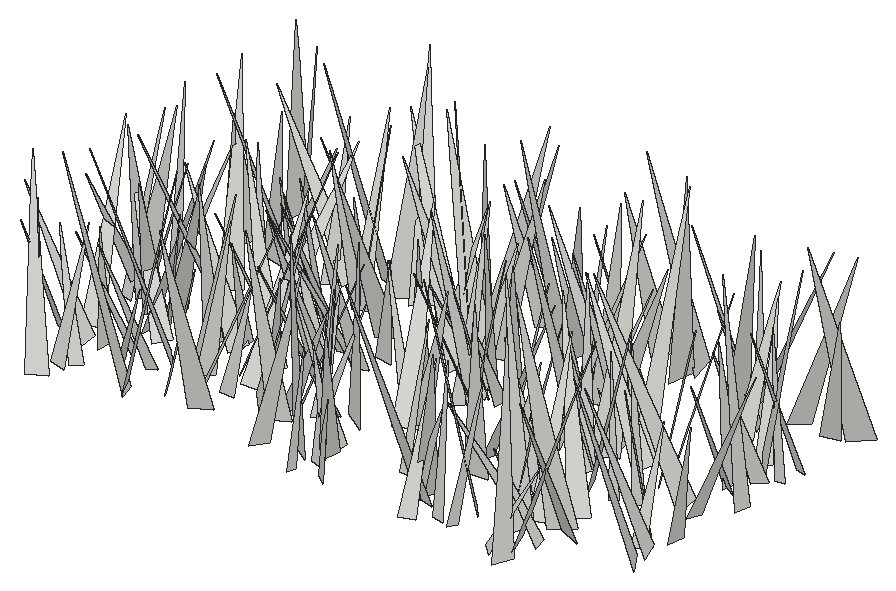
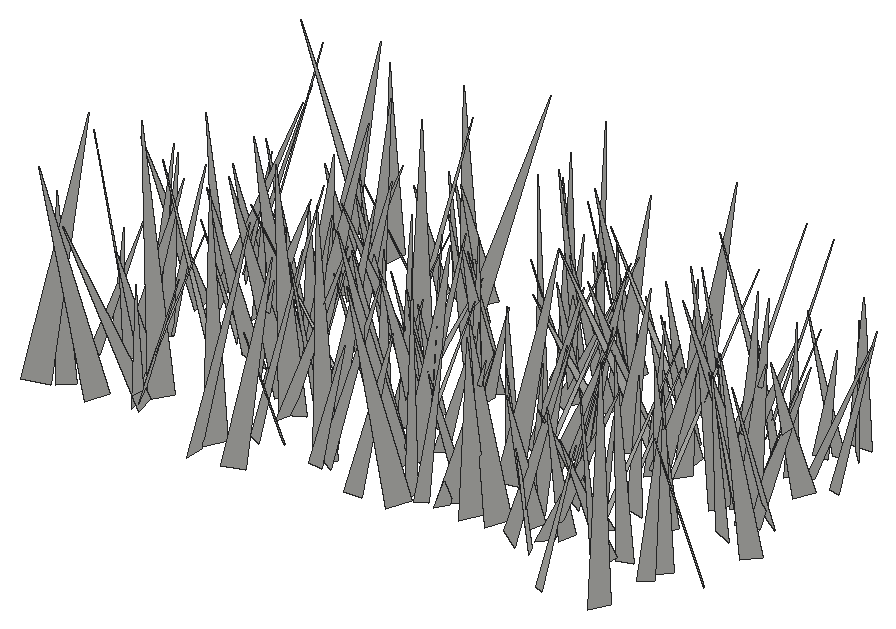
# SketchUp Ruby script. Lengths in inches.
U = 1.inch
M = Sketchup.active_model
def pt(a) = Geom::Point3d.new(a.map { |v| v * U })
def face(e, loops, mat)
  f = e.add_face(loops[0].map { |a| pt(a) })
  loops[1..].each { |l| e.add_face(l.map { |a| pt(a) }).erase! }
  f.material = f.back_material = mat if mat
  f
end
# faces: each face lists its corners as indices into pts; further lists are holes
def faces(e, pts, list, mat = nil) = list.each { |f| face(e, (f[0].is_a?(Array) ? f : [f]).map { |l| l.map { |i| pts[i] } }, mat) }
# xy, xz, yz: faces in a plane at the given z, y or x. An outline is a flat list of corners, or four numbers for a rectangle; further outlines are holes
def ring(l) = l.size == 4 ? [[l[0], l[1]], [l[2], l[1]], [l[2], l[3]], [l[0], l[3]]] : l.each_slice(2).to_a
def flat(e, list, mat, &to3) = list.each { |f| face(e, (f[0].is_a?(Array) ? f : [f]).map { |l| ring(l).map { |u, v| to3.(u, v) } }, mat) }
def xy(e, z, list, mat = nil) = flat(e, list, mat) { |x, y| [x, y, z] }
def xz(e, y, list, mat = nil) = flat(e, list, mat) { |x, z| [x, y, z] }
def yz(e, x, list, mat = nil) = flat(e, list, mat) { |y, z| [x, y, z] }
def lines(e, pts, list) = list.each { |a, b| e.add_line(pt(pts[a]), pt(pts[b])) }
# prism: a flat outline (further loops are holes) pulled along v
def prism(e, loops, v, mat = nil)
  f = face(e, loops, mat); d = Geom::Vector3d.new(v.map { |x| x * U })
  f.pushpull(f.normal.samedirection?(d) ? d.length : -d.length)
end
def box(e, o, s, mat = nil) = prism(e, [[o, [o[0] + s[0], o[1], o[2]], [o[0] + s[0], o[1] + s[1], o[2]], [o[0], o[1] + s[1], o[2]]]], [0, 0, s[2]], mat)
def at(x, y, z, deg = 0) = Geom::Transformation.translation(pt([x, y, z])) * Geom::Transformation.rotation(ORIGIN, Z_AXIS, deg.degrees)
def axes(o, x, y, z) = Geom::Transformation.new([*x, 0, *y, 0, *z, 0, *pt(o).to_a, 1])
def part(name) = M.definitions.add(name)
# library, detail: a bought-in or finely detailed component or shape, given as its bounding box
def library(name, o, s) = part(name).tap { |d| box(d.entities, o, s) }
def detail(e, o, s) = box(e.add_group.entities, o, s)
def put(e, d, t, mat = nil) = e.add_instance(d, t).tap { |i| i.material = mat if mat }
def group(e, t, mat = nil) = e.add_group.tap { |g| g.transformation = t; g.material = mat if mat }.entities
root = M.entities
c1 = part("fur_instance\#9")
p = [[0.8125,0,1.79],[0.67,-0.02,1.48],[0,-0.11,0],[0,0.11,0]]
faces(c1.entities,p,[[0,1,2,3]])
put(root,c1,axes([541.56,330.53,-21.66],[-6.82221,1.72842,2.33339],[1.55801,7.20655,-0.7829],[2.45045,0.23004,6.99407]))
put(root,c1,axes([539.97,331.04,-21.66],[2.36408,2.77163,0.06713],[2.67068,-2.25294,-1.03299],[0.74428,-0.71945,3.49339]))
put(root,c1,axes([533.52,333.23,-21.66],[-2.92587,-7.18113,1.16279],[-7.26033,2.80394,-0.95233],[-0.45638,1.43204,7.69561]))
put(root,c1,axes([533.1875,333.78,-21.66],[6.03142,-3.81553,0.06105],[-3.78285,-5.99326,-0.84318],[-0.50203,-0.68018,7.08699]))
put(root,c1,axes([516.45,333.74,-21.66],[2.5513,-6.67742,1.15565],[-6.68995,-2.67869,-0.70836],[-1.08074,0.81812,7.11304]))
put(root,c1,axes([525.87,333.9375,-21.66],[5.72206,-2.67718,0.30846],[-2.55509,-5.6197,-1.37653],[-0.85672,-1.12072,6.16558]))
put(root,c1,axes([525.14,331.34,-21.66],[-3.53887,0.08812,1.47041],[-0.2173,3.75324,-0.74791],[1.45693,0.77383,3.46005]))
put(root,c1,axes([541.94,333.51,-21.66],[-3.71284,-0.24914,0.82183],[0.046,3.58403,1.29433],[0.85753,-1.27095,3.48884]))
put(root,c1,axes([527.2,331.49,-21.66],[3.68214,4.39884,2.0354],[4.4735,-4.06815,0.69917],[-1.86561,-1.07294,5.69378]))
put(root,c1,axes([542.73,335.26,-21.66],[-1.67702,-6.45132,0.05531],[-6.32349,1.655,1.30744],[1.27907,-0.27646,6.53625]))
put(root,c1,axes([532.82,333.23,-21.66],[2.13927,-3.81253,0.27989],[-3.71667,-1.99926,1.17453],[0.89447,0.81104,4.21098]))
put(root,c1,axes([524.15,333.3,-21.66],[3.79237,5.90894,3.79832],[6.9076,-3.92109,-0.79686],[-1.27587,-3.6653,6.97586]))
put(root,c1,axes([533.98,331.07,-21.66],[-3.10832,3.75001,0.92239],[3.63037,3.24121,-0.94342],[1.31674,-0.08395,4.77852]))
put(root,c1,axes([506.01,331.8,-21.66],[2.91004,3.86675,2.0314],[3.84438,-3.42612,1.0144],[-2.0734,-0.92551,4.73192]))
put(root,c1,axes([506.5,330.92,-21.66],[-2.09458,6.39775,0.76013],[6.40195,1.97698,1.00139],[-0.72385,-1.02792,6.657]))
put(root,c1,axes([511.85,332.63,-21.66],[-7.0839,-2.86843,1.00142],[-2.98784,7.03787,-0.97651],[0.55097,1.28563,7.57997]))
put(root,c1,axes([540.91,332.69,-21.66],[7.89024,2.57718,0.73013],[2.64489,-7.85516,-0.85554],[-0.42369,-1.04189,8.25626]))
put(root,c1,axes([535.51,332.02,-21.66],[1.56469,4.5597,1.40699],[4.65343,-1.78584,0.61247],[-1.05645,-1.11294,4.78163]))
put(root,c1,axes([521.78,332.56,-21.66],[5.79665,-1.91222,1.6292],[-2.17494,-5.87047,0.84811],[-1.25719,1.33905,6.04471]))
put(root,c1,axes([506.71,332.58,-21.66],[0.82444,4.69785,1.50621],[4.90559,-0.61872,-0.75536],[0.52313,-1.60174,4.70945]))
put(root,c1,axes([536.58,332.05,-21.66],[-4.01234,0.85775,1.7856],[0.34464,4.27421,-1.27879],[1.95072,1.00913,3.89863]))
put(root,c1,axes([547.68,335.24,-21.66],[-5.81163,-3.8947,1.27527],[-3.71182,5.94036,1.22659],[1.73708,-0.33677,6.88761]))
put(root,c1,axes([525.62,334.3,-21.66],[3.23004,-2.47849,1.2151],[-2.38486,-3.44753,-0.69249],[-1.3899,0.15559,4.01205]))
put(root,c1,axes([513.48,334.33,-21.66],[4.61843,1.91697,0.98697],[2.11588,-4.47821,-1.2031],[-0.41467,-1.49987,4.85358]))
put(root,c1,axes([507.57,333.29,-21.66],[-1.66438,3.94539,0.96796],[4.04045,1.49913,0.83702],[-0.42169,-1.20819,4.19948]))
put(root,c1,axes([526.01,332.76,-21.66],[2.58836,6.22661,1.98748],[6.38761,-2.86286,0.6503],[-1.38536,-1.56644,6.71174]))
put(root,c1,axes([511.66,332.62,-21.66],[6.24718,3.3719,1.68528],[3.2403,-6.4703,0.93425],[-1.92623,0.05148,7.03734]))
put(root,c1,axes([504.36,336,-21.66],[-1.82022,-4.66244,0.24993],[-4.60062,1.83672,0.75812],[0.79693,-0.04591,4.9474]))
put(root,c1,axes([536.6875,334.27,-21.66],[-5.72763,-4.55632,1.57593],[-4.80185,5.61014,-1.23206],[0.43111,1.95337,7.21442]))
put(root,c1,axes([509.44,335.03,-21.66],[3.62629,-0.3933,0.08931],[-0.3696,-3.56406,-0.68808],[-0.16141,-0.67481,3.58206]))
put(root,c1,axes([520.99,335.46,-21.66],[1.6386,-6.2759,2.07036],[-6.47654,-1.94928,-0.78297],[-1.31443,1.78093,6.43885]))
put(root,c1,axes([541.84,335.72,-21.66],[2.92408,-7.38877,2.72238],[-7.56214,-3.44459,-1.22649],[-2.19528,2.02396,7.85111]))
put(root,c1,axes([511.32,335.62,-21.66],[-0.67131,-4.1889,0.93111],[-4.10147,0.34927,-1.38579],[-1.26165,1.09345,4.00962]))
put(root,c1,axes([547.5,336.76,-21.66],[-5.8236,-1.97497,1.08531],[-1.72724,5.8434,1.36532],[1.44743,-0.9731,5.99589]))
put(root,c1,axes([509.05,336.7,-21.66],[-4.05728,-2.523,0.42943],[-2.40041,4.03064,1.00168],[0.88766,-0.63233,4.67158]))
put(root,c1,axes([511.47,337.29,-21.66],[-5.81753,-5.50464,0.89808],[-5.45533,5.88597,0.73893],[1.16061,0.07452,7.97488]))
put(root,c1,axes([507.45,336.1,-21.66],[4.3427,-1.50818,1.19732],[-1.3579,-4.49272,-0.73402],[-1.36538,-0.32877,4.53816]))
put(root,c1,axes([540.08,334.25,-21.66],[-7.50799,1.69583,1.59774],[1.55933,7.66276,-0.80567],[1.73121,0.45255,7.65484]))
put(root,c1,axes([506.3,335.9375,-21.66],[-5.398,0.07669,0.31538],[0.11355,5.36878,0.63804],[0.30406,-0.64352,5.36071]))
put(root,c1,axes([525.82,335.21,-21.66],[-5.12979,-1.0122,0.11272],[-1.018,5.07872,-0.72273],[-0.03042,0.73083,5.17851]))
put(root,c1,axes([538.33,335.78,-21.66],[3.90059,1.73334,0.99556],[1.91928,-3.85762,-0.80331],[-0.55855,-1.15086,4.19211]))
put(root,c1,axes([516.6,335.97,-21.66],[-0.37702,3.57753,2.02822],[3.88687,0.97529,-0.99777],[1.34335,-1.81786,3.4562]))
put(root,c1,axes([520.51,336.86,-21.66],[3.4493,-3.36014,0.02886],[-3.29462,-3.37365,0.97621],[0.66096,0.719,4.71542]))
put(root,c1,axes([535.66,337.69,-21.66],[-3.34335,-1.51871,0.13226],[-1.40215,3.18862,1.16988],[0.59829,-1.01398,3.48078]))
put(root,c1,axes([533.93,337.52,-21.66],[1.85268,-6.56464,1.39244],[-6.70428,-1.74747,0.68181],[0.2934,1.52239,6.78691]))
put(root,c1,axes([518.4,337.87,-21.66],[5.40312,-1.02873,0.51523],[-0.87968,-5.28821,-1.33359],[-0.74156,-1.2223,5.33606]))
put(root,c1,axes([514.91,335.92,-21.66],[6.15209,3.35933,0.33959],[3.37614,-6.1107,-0.71393],[0.04606,-0.78923,6.97306]))
put(root,c1,axes([523.08,338.05,-21.66],[-1.88046,-5.21634,0.33238],[-5.10911,1.75978,-1.28722],[-1.10347,0.74146,5.39346]))
put(root,c1,axes([518.49,336.52,-21.66],[5.36031,4.39922,1.5205],[4.6383,-5.24227,-1.18439],[-0.38885,-1.88772,6.83252]))
put(root,c1,axes([530.55,335.12,-21.66],[1.48106,4.37962,0.44895],[4.22706,-1.54701,1.14671],[-1.23071,-0.04293,4.4788]))
put(root,c1,axes([524.4,338.14,-21.66],[-2.31612,-6.1908,2.36322],[-6.27799,2.85121,1.3163],[2.12077,1.67923,6.47748]))
put(root,c1,axes([522.84,336.87,-21.66],[2.35379,3.88662,0.95748],[3.9563,-2.09005,-1.24191],[0.60851,-1.44527,4.3708]))
put(root,c1,axes([514.25,337.01,-21.66],[4.29417,-2.87763,1.75823],[-3.19183,-4.38696,0.6155],[-1.08829,1.5119,5.13243]))
put(root,c1,axes([540.23,335.51,-21.66],[-3.17134,4.85922,0.78552],[4.77597,3.26378,-0.90795],[1.19131,-0.14895,5.73106]))
put(root,c1,axes([546.72,336.72,-21.66],[-2.21972,3.26489,1.22418],[3.2229,2.47495,-0.75684],[1.3308,-0.54808,3.87477]))
put(root,c1,axes([547.09,337.51,-21.66],[2.56501,3.25674,2.5986],[3.3721,-3.41499,0.95138],[-2.44704,-1.29222,4.03491]))
put(root,c1,axes([547.91,338.72,-21.66],[4.83385,-1.43847,0.54232],[-1.36908,-4.84202,-0.64023],[-0.69925,-0.46374,5.00254]))
put(root,c1,axes([522.52,337.2,-21.66],[-2.57998,2.99071,1.64125],[3.02202,2.95835,-0.64026],[1.58287,-0.77341,3.89753]))
put(root,c1,axes([538,338.5625,-21.66],[-4.52682,2.09063,1.69581],[2.46981,4.54531,0.98938],[1.07078,-1.64562,4.88712]))
put(root,c1,axes([535.84,337.99,-21.66],[1.71183,-4.04593,1.56999],[-4.29437,-1.33542,1.2409],[0.62675,1.9005,4.21427]))
put(root,c1,axes([507.27,340.95,-21.66],[4.70982,-4.44224,0.12242],[-4.38661,-4.67586,-0.90827],[-0.71149,-0.57769,6.41023]))
put(root,c1,axes([541.74,337.39,-21.66],[-2.77056,6.19265,0.76015],[6.19361,2.62958,1.15202],[-0.75223,-1.15721,6.68563]))
put(root,c1,axes([512.31,340.11,-21.66],[5.42089,-2.3865,1.81758],[-2.19868,-5.71457,-0.94576],[-2.04078,-0.18248,5.84696]))
put(root,c1,axes([521.05,337.22,-21.66],[4.24517,2.47398,0.29086],[2.34061,-4.15824,1.20716],[-0.85248,0.90284,4.76286]))
put(root,c1,axes([512.71,338.43,-21.66],[5.08359,-0.28901,1.82683],[-0.68576,-5.25683,1.07667],[-1.71772,1.24337,4.97667]))
put(root,c1,axes([527.8,339.99,-21.66],[3.51302,-4.23345,1.0034],[-4.35037,-3.40123,0.88101],[0.05668,1.33409,5.43021]))
put(root,c1,axes([509.77,338.5625,-21.66],[-3.53792,4.34861,0.23075],[4.30519,3.44804,1.02808],[-0.65501,-0.82532,5.51093]))
put(root,c1,axes([517.29,337.51,-21.66],[-1.69129,6.09931,0.73665],[6.01995,1.79783,-1.06428],[1.22654,-0.41345,6.23934]))
put(root,c1,axes([513.87,341.21,-21.66],[4.34393,-1.36952,0.92271],[-1.07858,-4.31928,-1.3331],[-1.25046,-1.03195,4.35524]))
put(root,c1,axes([508.99,340.11,-21.66],[3.83115,1.46002,1.29175],[1.69697,-3.89964,-0.62537],[-0.95945,-1.06731,4.05194]))
put(root,c1,axes([512.04,342.14,-21.66],[-5.96811,-4.81477,0.42538],[-4.75156,5.96808,0.88657],[0.88638,-0.42578,7.61672]))
put(root,c1,axes([505.45,337.41,-21.66],[-4.47188,4.60163,0.40246],[4.4512,4.44255,-1.33612],[1.23441,0.65071,6.27595]))
put(root,c1,axes([508.34,341.62,-21.66],[6.88515,-2.28469,0.18682],[-2.24647,-6.84269,-0.88939],[-0.45618,-0.78602,7.19959]))
put(root,c1,axes([505.62,342.13,-21.66],[0.74185,-5.118,0.35857],[-5.01336,-0.80012,-1.04825],[-1.09027,0.19676,5.06413]))
put(root,c1,axes([508.27,339.13,-21.66],[6.55283,1.12937,1.12544],[0.97488,-6.60494,0.95181],[-1.26162,0.76214,6.58096]))
put(root,c1,axes([518.27,342.4,-21.66],[1.50349,-5.86365,0.5049],[-5.82358,-1.55753,-0.74685],[-0.85041,0.2992,6.00709]))
put(root,c1,axes([540.07,340.5,-21.66],[5.73054,2.09287,1.0832],[2.24178,-5.71944,-0.8093],[-0.7265,-1.14039,6.04684]))
put(root,c1,axes([513.75,340.67,-21.66],[-5.32926,2.77314,1.19327],[2.9808,5.21718,1.1879],[0.47858,-1.6143,5.88899]))
put(root,c1,axes([505.83,342.23,-21.66],[4.78165,-4.93816,1.39024],[-4.88475,-4.96331,-0.82896],[-1.56762,0.40313,6.82367]))
put(root,c1,axes([533.17,339.55,-21.66],[5.62442,0.34622,0.61815],[0.22701,-5.5658,1.05184],[-0.67115,1.01884,5.53603]))
put(root,c1,axes([515.5625,338.77,-21.66],[6.75975,3.62956,0.52461],[3.54067,-6.74583,1.04905],[-0.95528,0.68056,7.60048]))
put(root,c1,axes([519.79,343.73,-21.66],[-4.86076,-4.47494,0.06756],[-4.36579,4.76306,1.38194],[0.98465,-0.972,6.46083]))
put(root,c1,axes([516.86,340.05,-21.66],[-4.60264,5.20733,0.96805],[5.29634,4.53648,0.77902],[0.04773,-1.24166,6.90606]))
put(root,c1,axes([545.83,342.34,-21.66],[-8.03194,-0.35365,0.82088],[-0.22203,7.97883,1.26494],[0.86581,-1.23463,7.93959]))
put(root,c1,axes([538.1,342.38,-21.66],[-1.48143,-7.59825,2.03928],[-7.84224,1.26126,-0.99758],[-0.62555,2.18232,7.67677]))
put(root,c1,axes([526.82,340.23,-21.66],[-4.67353,1.04438,0.03845],[1.02272,4.60667,-0.8165],[0.21505,0.78861,4.71868]))
put(root,c1,axes([543.59,340.64,-21.66],[-4.82421,0.67017,1.12309],[0.52178,4.9221,-0.69578],[1.19925,0.5543,4.82058]))
put(root,c1,axes([542.04,340.23,-21.66],[0.68638,4.30492,0.85677],[4.11958,-0.93113,1.37825],[-1.51508,-0.58153,4.13569]))
put(root,c1,axes([527.17,339.36,-21.66],[-3.85678,5.81728,0.33644],[5.7739,3.8696,-0.71896],[0.78484,0.11882,6.94252]))
put(root,c1,axes([530.33,342.53,-21.66],[-3.6362,-3.51378,0.23491],[-3.4583,3.49912,-1.19165],[-0.6648,1.01649,4.91412]))
put(root,c1,axes([520.81,343.1875,-21.66],[-0.18696,-5.47828,1.21386],[-5.53827,-0.01495,-0.92048],[-0.90141,1.22808,5.40363]))
put(root,c1,axes([546.94,341.67,-21.66],[5.55155,-0.72144,0.45458],[-0.77671,-5.51397,0.73462],[-0.35191,0.78896,5.54982]))
put(root,c1,axes([513.29,344.1,-21.66],[-3.4189,-2.83051,0.24342],[-2.77437,3.40847,0.66713],[0.61145,-0.36118,4.38812]))
put(root,c1,axes([537.24,344.0625,-21.66],[4.28198,-1.79299,1.3249],[-1.43721,-4.41332,-1.32759],[-1.70429,-0.78312,4.44833]))
put(root,c1,axes([537.33,342.74,-21.66],[-3.51582,-2.14374,0.80605],[-2.26912,3.46073,-0.69338],[0.31056,1.01688,4.05904]))
put(root,c1,axes([524.47,344.43,-21.66],[-0.27546,-6.0552,1.07535],[-6.00995,0.49341,1.23885],[1.30474,0.99438,5.93351]))
put(root,c1,axes([538.68,341.87,-21.66],[-5.6137,1.8249,1.28834],[1.63706,5.7317,-0.98561],[1.51991,0.56669,5.82001]))
put(root,c1,axes([517.29,343.69,-21.66],[-3.50463,1.38607,1.3282],[1.66931,3.56562,0.68373],[0.94799,-1.15452,3.70623]))
put(root,c1,axes([504.88,341.3,-21.66],[2.36342,5.34352,0.74133],[5.25737,-2.46286,0.99138],[-1.20944,-0.26392,5.75813]))
put(root,c1,axes([504.83,343.83,-21.66],[4.88196,1.64498,0.71636],[1.77456,-4.73338,-1.22423],[-0.26474,-1.39349,5.00407]))
put(root,c1,axes([546.35,345.47,-21.66],[-1.70648,-4.83175,0.15849],[-4.67215,1.69151,1.26205],[1.24174,-0.27565,4.96639]))
put(root,c1,axes([518.73,344.09,-21.66],[-1.8038,-4.78632,0.84713],[-4.75617,1.55162,-1.36069],[-1.00264,1.25053,4.93062]))
put(root,c1,axes([529.75,345.1,-21.66],[2.79879,-2.29313,0.37979],[-2.08936,-2.74248,-1.16161],[-1.01846,-0.6755,3.42672]))
put(root,c1,axes([533.73,342.74,-21.66],[3.61402,1.40651,0.81578],[1.29809,-3.69316,0.61679],[-0.97915,0.29527,3.8287]))
put(root,c1,axes([528.375,344.39,-21.66],[-6.31827,-0.38458,1.65434],[-0.20418,6.49842,0.73085],[1.68614,-0.65417,6.28763]))
put(root,c1,axes([521.23,344.8125,-21.66],[0.93641,-4.49496,0.58968],[-4.44892,-0.79539,1.00188],[0.87152,0.76939,4.48082]))
put(root,c1,axes([529.68,342.41,-21.66],[4.20978,2.5999,1.29958],[2.36123,-4.39284,1.13935],[-1.69498,0.33775,4.81493]))
put(root,c1,axes([528.42,345.37,-21.66],[-1.9531,-3.93926,0.49775],[-3.87343,2.01224,0.72636],[0.87298,0.11511,4.33645]))
put(root,c1,axes([516.32,345.5,-21.66],[-3.7934,-3.57067,0.95546],[-3.47781,3.9116,0.81037],[1.25196,0.04698,5.14615]))
put(root,c1,axes([541.03,344.29,-21.66],[-5.49496,2.98551,0.84144],[3.09795,5.36781,1.18541],[0.15494,-1.44541,6.14025]))
put(root,c1,axes([528.74,345.63,-21.66],[-1.97091,-5.99186,1.73382],[-5.97714,2.33419,1.27215],[1.7839,1.20092,6.17807]))
put(root,c1,axes([519.7,347.12,-21.66],[2.52782,-6.77606,0.30453],[-6.73549,-2.54598,-0.74076],[-0.80053,0.02468,7.19418]))
put(root,c1,axes([527.9,343.41,-21.66],[3.76541,-0.98312,2.37268],[-1.72485,-4.08783,1.04352],[-1.9029,1.75998,3.74912]))
put(root,c1,axes([503.2,345.1875,-21.66],[2.93008,-5.46925,1.49234],[-5.65269,-2.69042,1.23848],[0.43226,1.89052,6.07982]))
put(root,c1,axes([546.32,345.91,-21.66],[5.03393,-2.19184,1.50174],[-1.99616,-5.24318,-0.96135],[-1.75349,-0.32355,5.40559]))
put(root,c1,axes([543.01,343.3,-21.66],[3.77893,2.89431,1.05154],[2.64296,-3.90266,1.24382],[-1.58036,0.3941,4.59459]))
put(root,c1,axes([538.375,346.19,-21.66],[-6.39849,-1.36399,1.46981],[-1.16574,6.52941,0.98452],[1.63152,-0.68393,6.46776]))
put(root,c1,axes([526.34,347.17,-21.66],[-3.05725,-3.63504,0.09512],[-3.51202,2.98398,1.15363],[0.94245,-0.67208,4.60753]))
put(root,c1,axes([548.6,344.05,-21.66],[-7.01031,-0.43579,1.43561],[-0.72042,6.99511,-1.39453],[1.31601,1.50792,6.88401]))
put(root,c1,axes([506.15,344.17,-21.66],[1.54209,5.92638,1.72605],[6.04197,-1.81335,0.82809],[-1.2633,-1.43843,6.06748]))
put(root,c1,axes([538.4,343.94,-21.66],[-4.94866,6.16749,2.69055],[6.18584,5.48419,-1.19385],[2.6481,-1.28527,7.81677]))
put(root,c1,axes([528.09,344.72,-21.66],[-2.58112,4.19595,2.18678],[4.13957,3.20902,-1.27135],[2.29171,-1.07069,4.75939]))
put(root,c1,axes([547.41,347.16,-21.66],[1.87791,-4.76016,0.94457],[-4.63856,-2.05833,-1.15104],[-1.42657,0.4266,4.98606]))
put(root,c1,axes([528.99,347.16,-21.66],[4.92449,-2.5321,0.51516],[-2.43841,-4.92066,-0.87679],[-0.85503,-0.55051,5.46748]))
put(root,c1,axes([522.125,346.92,-21.66],[0.84886,-4.32385,0.54485],[-4.30912,-0.7498,0.76315],[0.65118,0.6747,4.3398]))
put(root,c1,axes([511.91,345.19,-21.66],[-0.00345,4.9845,1.60202],[5.18158,-0.22632,0.71534],[-0.75028,-1.58596,4.93291]))
put(root,c1,axes([535.35,343.38,-21.66],[4.61833,5.37447,0.17353],[5.34108,-4.61135,0.67253],[-0.62281,0.30742,7.05419]))
put(root,c1,axes([527.52,344.41,-21.66],[0.92539,5.82013,0.73982],[5.78512,-1.02986,0.86568],[-0.97656,-0.58571,5.82931]))
put(root,c1,axes([530.06,346.56,-21.66],[3.37975,2.64749,1.02841],[2.82915,-3.2791,-0.85611],[-0.25046,-1.31446,4.20701]))
put(root,c1,axes([539.36,346.29,-21.66],[-2.08975,2.94897,0.92989],[3.09202,1.98432,0.65582],[-0.0238,-1.13764,3.55435]))
put(root,c1,axes([525.2,346.6,-21.66],[-3.9914,1.89648,0.82188],[2.01712,3.964,0.64912],[0.45094,-0.94526,4.3711]))
put(root,c1,axes([536.39,346.9,-21.66],[5.35038,-4.23141,0.69897],[-4.27634,-5.17862,1.38378],[0.32603,1.51562,6.67957]))
put(root,c1,axes([513.27,346.45,-21.66],[-1.82115,-3.36265,1.61921],[-3.73204,1.65736,-0.7556],[0.03439,1.7865,3.74875]))
put(root,c1,axes([515.16,346.69,-21.66],[-1.86227,-3.58892,1.59018],[-3.91628,1.57852,-1.02377],[-0.26793,1.87217,3.91156]))
put(root,c1,axes([541.4375,347.21,-21.66],[5.88028,2.97965,0.94292],[3.11911,-5.72141,-1.37172],[-0.19635,-1.65292,6.44782]))
put(root,c1,axes([511.94,348.58,-21.66],[-5.99234,-4.15881,0.58341],[-4.19764,5.96205,-0.6148],[0.12593,0.83815,7.26814]))
put(root,c1,axes([509.05,345.8,-21.66],[-5.83364,4.02968,1.05878],[3.90844,5.92385,-1.01134],[1.44341,0.24573,7.01761]))
put(root,c1,axes([534.62,348.62,-21.66],[2.7668,-7.06079,2.0724],[-7.35623,-2.5972,0.97226],[0.18857,2.28135,7.52095]))
put(root,c1,axes([516.43,348.72,-21.66],[0.40641,-5.35004,1.66525],[-5.54368,-0.62666,-0.66032],[-0.81458,1.59547,5.32467]))
put(root,c1,axes([516.32,349.23,-21.66],[4.42301,-0.66017,1.25029],[-0.31732,-4.46498,-1.23502],[-1.37781,-1.09094,4.29808]))
put(root,c1,axes([540.4,344.97,-21.66],[0.71123,8.26754,0.30404],[8.18462,-0.74766,1.1847],[-1.20692,-0.19821,8.21307]))
put(root,c1,axes([523.04,347.84,-21.66],[2.00403,4.77087,1.2081],[4.88814,-1.77806,-1.08691],[0.57161,-1.52123,5.05925]))
put(root,c1,axes([534.01,347.0625,-21.66],[2.59525,5.12132,1.23508],[5.09738,-2.78884,0.85303],[-1.33041,-0.69505,5.67763]))
put(root,c1,axes([506.05,349.76,-21.66],[5.02867,-2.50397,0.95955],[-2.41233,-5.11484,-0.70513],[-1.17101,-0.21602,5.57317]))
put(root,c1,axes([534.87,349.08,-21.66],[-6.53044,0.59698,0.86107],[0.69842,6.53195,0.76827],[0.78105,-0.84949,6.51251]))
put(root,c1,axes([525.59,348.375,-21.66],[-4.55755,6.1935,2.40469],[6.62517,4.45559,1.08074],[0.49905,-2.58872,7.61332]))
put(root,c1,axes([524.87,348.28,-21.66],[-5.85102,-5.01294,3.05498],[-5.59861,6.06235,-0.77491],[1.76582,2.61061,7.66574]))
put(root,c1,axes([546.52,348.53,-21.66],[-3.91032,-4.73518,3.93684],[-5.20514,5.03349,0.88414],[3.29046,2.33522,6.07707]))
put(root,c1,axes([548.22,347.98,-21.66],[0.93593,4.40998,1.37185],[4.37962,-1.29175,1.16453],[-1.46587,-1.0437,4.3552]))
put(root,c1,axes([548.48,349.64,-21.66],[-2.25031,-4.2676,0.76277],[-4.32128,2.13921,-0.77999],[-0.34742,1.03417,4.76108]))
put(root,c1,axes([508.67,350.09,-21.66],[0.4901,-6.09421,1.40714],[-6.12992,-0.18765,1.32232],[1.24239,1.47818,5.96918]))
put(root,c1,axes([530.84,350.21,-21.66],[-1.51779,-7.89387,2.17922],[-8.18213,1.37007,-0.73587],[-0.33897,2.275,8.00471]))
put(root,c1,axes([526.27,349.11,-21.66],[4.89354,-4.52263,1.72188],[-4.82903,-4.72322,1.31813],[-0.31551,2.14541,6.53173]))
put(root,c1,axes([529.74,351.7,-21.66],[6.8807,-3.2851,0.24825],[-3.20439,-6.80705,-1.26238],[-0.76512,-1.03432,7.51946]))
put(root,c1,axes([503.4,349.42,-21.66],[3.56732,3.05528,0.6125],[3.0981,-3.37772,-1.19517],[0.33415,-1.30074,4.54225]))
put(root,c1,axes([511.95,347.73,-21.66],[-0.74484,5.04348,0.31723],[4.84937,0.80355,-1.38926],[1.42161,-0.09859,4.90524]))
put(root,c1,axes([506.35,351.0625,-21.66],[4.04472,-2.80495,1.23292],[-2.68281,-4.22845,-0.81868],[-1.47998,-0.00072,4.85358]))
put(root,c1,axes([525.9,349.37,-21.66],[7.69259,-0.4984,1.40276],[-0.64413,-7.77059,0.77146],[-1.3421,0.87272,7.67002]))
put(root,c1,axes([541.98,351.69,-21.66],[7.73764,-3.02475,0.93063],[-2.93122,-7.77665,-0.90436],[-1.19293,-0.51074,8.25847]))
put(root,c1,axes([534.57,352.23,-21.66],[-3.08937,-5.14938,0.76665],[-5.09175,3.1744,0.80332],[1.08532,0.23487,5.95105]))
put(root,c1,axes([522.34,351.96,-21.66],[3.93846,-2.19121,0.70559],[-1.95473,-3.92185,-1.26841],[-1.21585,-0.79274,4.32481]))
put(root,c1,axes([529.62,351.84,-21.66],[-2.67742,-5.68655,1.10676],[-5.79247,2.6077,-0.61446],[-0.09527,1.2623,6.25523]))
put(root,c1,axes([546.22,349,-21.66],[-4.08982,2.78235,0.32679],[2.66533,4.04258,-1.06229],[0.86271,0.7007,4.83111]))
put(root,c1,axes([513.89,351.03,-21.66],[-6.12139,2.10353,0.29479],[2.12072,6.0019,1.20952],[-0.1196,-1.23917,6.35872]))
put(root,c1,axes([521.13,351.56,-21.66],[-5.2528,1.04607,1.18822],[1.28573,5.22141,1.0871],[0.92359,-1.31932,5.24446]))
put(root,c1,axes([523.26,351.76,-21.66],[6.36794,0.62079,2.33056],[0.97414,-6.68136,-0.88201],[-2.20634,-1.15823,6.33704]))
put(root,c1,axes([513.05,349.99,-21.66],[-4.28711,2.60894,1.39768],[2.40918,4.50508,-1.01958],[1.71929,0.19268,4.91389]))
put(root,c1,axes([509.375,350.61,-21.66],[3.95352,-1.35205,0.74696],[-1.51739,-3.78343,1.18299],[-0.28899,1.3689,4.00736]))
put(root,c1,axes([515.64,352.17,-21.66],[-3.53449,-6.31522,1.62159],[-6.50822,3.306,-1.31053],[-0.39309,2.04757,7.11738]))
put(root,c1,axes([533,351.47,-21.66],[2.4928,2.63766,0.46244],[2.65596,-2.35455,-0.88721],[0.34203,-0.94022,3.51911]))
put(root,c1,axes([542.6,352.8,-21.66],[-3.61548,-1.81279,0.7212],[-1.71327,3.67656,0.65243],[0.9333,-0.2734,3.99152]))
put(root,c1,axes([529.875,352.4375,-21.66],[0.54062,-3.9189,1.26852],[-4.01221,-0.79056,-0.73238],[-0.93225,1.12979,3.88763]))
put(root,c1,axes([515.33,350.11,-21.66],[-4.48164,3.41054,1.04148],[3.17852,4.57879,-1.31654],[1.61662,0.45221,5.47573]))
put(root,c1,axes([543.35,350.66,-21.66],[-2.74828,4.07366,1.32335],[3.94461,3.01992,-1.10419],[1.66916,-0.42944,4.78838]))
put(root,c1,axes([521.12,351.04,-21.66],[-5.13567,3.95215,0.39173],[3.97037,5.09374,0.66187],[-0.09557,-0.76314,6.44644]))
put(root,c1,axes([513.79,352.49,-21.66],[4.93042,2.67254,1.54888],[2.99605,-4.84755,-1.1728],[-0.75178,-1.79146,5.48417]))
put(root,c1,axes([543.22,352.3,-21.66],[-5.70122,-3.26457,0.62497],[-3.32356,5.6155,-0.98593],[0.04408,1.16649,6.49533]))
put(root,c1,axes([548.85,354.78,-21.66],[4.03591,-7.21522,0.98619],[-7.10178,-4.1491,-1.2924],[-1.61145,0.21471,8.16564]))
put(root,c1,axes([547.27,353.88,-21.66],[2.80299,-5.03768,0.10257],[-5.00094,-2.76705,0.76127],[0.6159,0.45904,5.71449]))
put(root,c1,axes([517.29,351.15,-21.66],[5.828,-3.21448,3.45143],[-4.0564,-6.21538,1.06086],[-2.40642,2.69201,6.57061]))
put(root,c1,axes([526.02,353.77,-21.66],[1.56838,-4.91392,1.31708],[-4.91027,-1.82266,-0.95305],[-1.33063,0.93404,5.06933]))
put(root,c1,axes([509.39,351.99,-21.66],[-5.60874,-1.91132,2.91151],[-2.48414,6.06379,-0.80475],[2.44113,1.77916,5.87056]))
put(root,c1,axes([536.06,354.01,-21.66],[7.26083,-2.43104,1.92439],[-2.31077,-7.51014,-0.76873],[-2.06726,-0.14373,7.61831]))
put(root,c1,axes([523.2,352.98,-21.66],[5.70203,-3.94241,1.833],[-4.2894,-5.59456,1.31056],[-0.70959,2.13867,6.80721]))
put(root,c1,axes([518.92,351.4,-21.66],[5.10712,-2.96498,5.20518],[-4.57955,-6.3419,0.88079],[-3.86171,3.59957,5.83935]))
put(root,c1,axes([544.84,354.05,-21.66],[6.03076,-3.95506,0.64167],[-4.00583,-5.92637,1.12057],[0.08689,1.28836,7.12438]))
put(root,c1,axes([533.49,355.55,-21.66],[3.60817,-5.34608,1.25489],[-5.24687,-3.79935,-1.09972],[-1.62036,0.39817,6.35531]))
put(root,c1,axes([510.59,355.74,-21.66],[-2.24525,-3.81491,0.32062],[-3.67914,2.25292,1.04201],[1.05843,-0.26136,4.3022]))
put(root,c1,axes([506.52,355.21,-21.66],[7.00851,-2.19777,2.01204],[-2.01969,-7.2848,-0.92211],[-2.19075,-0.31499,7.28692]))
put(root,c1,axes([542.125,353,-21.66],[6.26365,0.83218,0.34032],[0.77044,-6.2027,0.98722],[-0.46342,0.93576,6.24109]))
put(root,c1,axes([542.62,353.07,-21.66],[-4.924,0.48292,1.1816],[0.20052,4.94285,-1.18453],[1.26062,1.10005,4.80373]))
put(root,c1,axes([536.34,355.62,-21.66],[-7.391,-1.41623,2.02124],[-1.14457,7.62073,1.15434],[2.18657,-0.79801,7.4364]))
